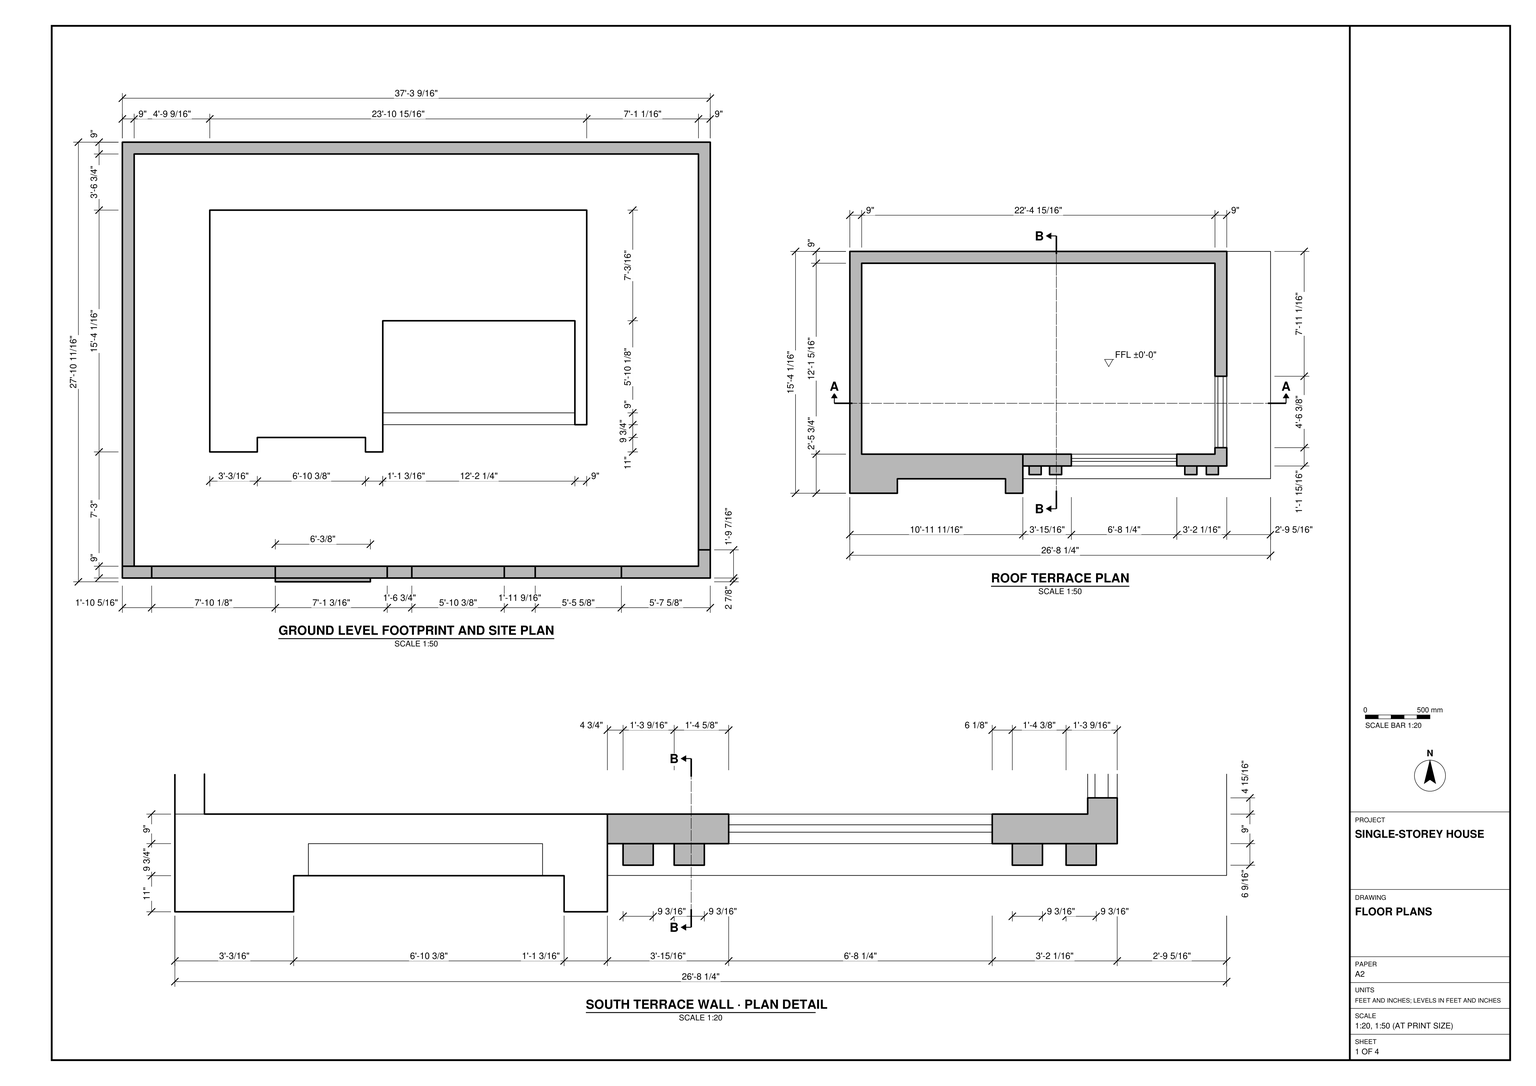
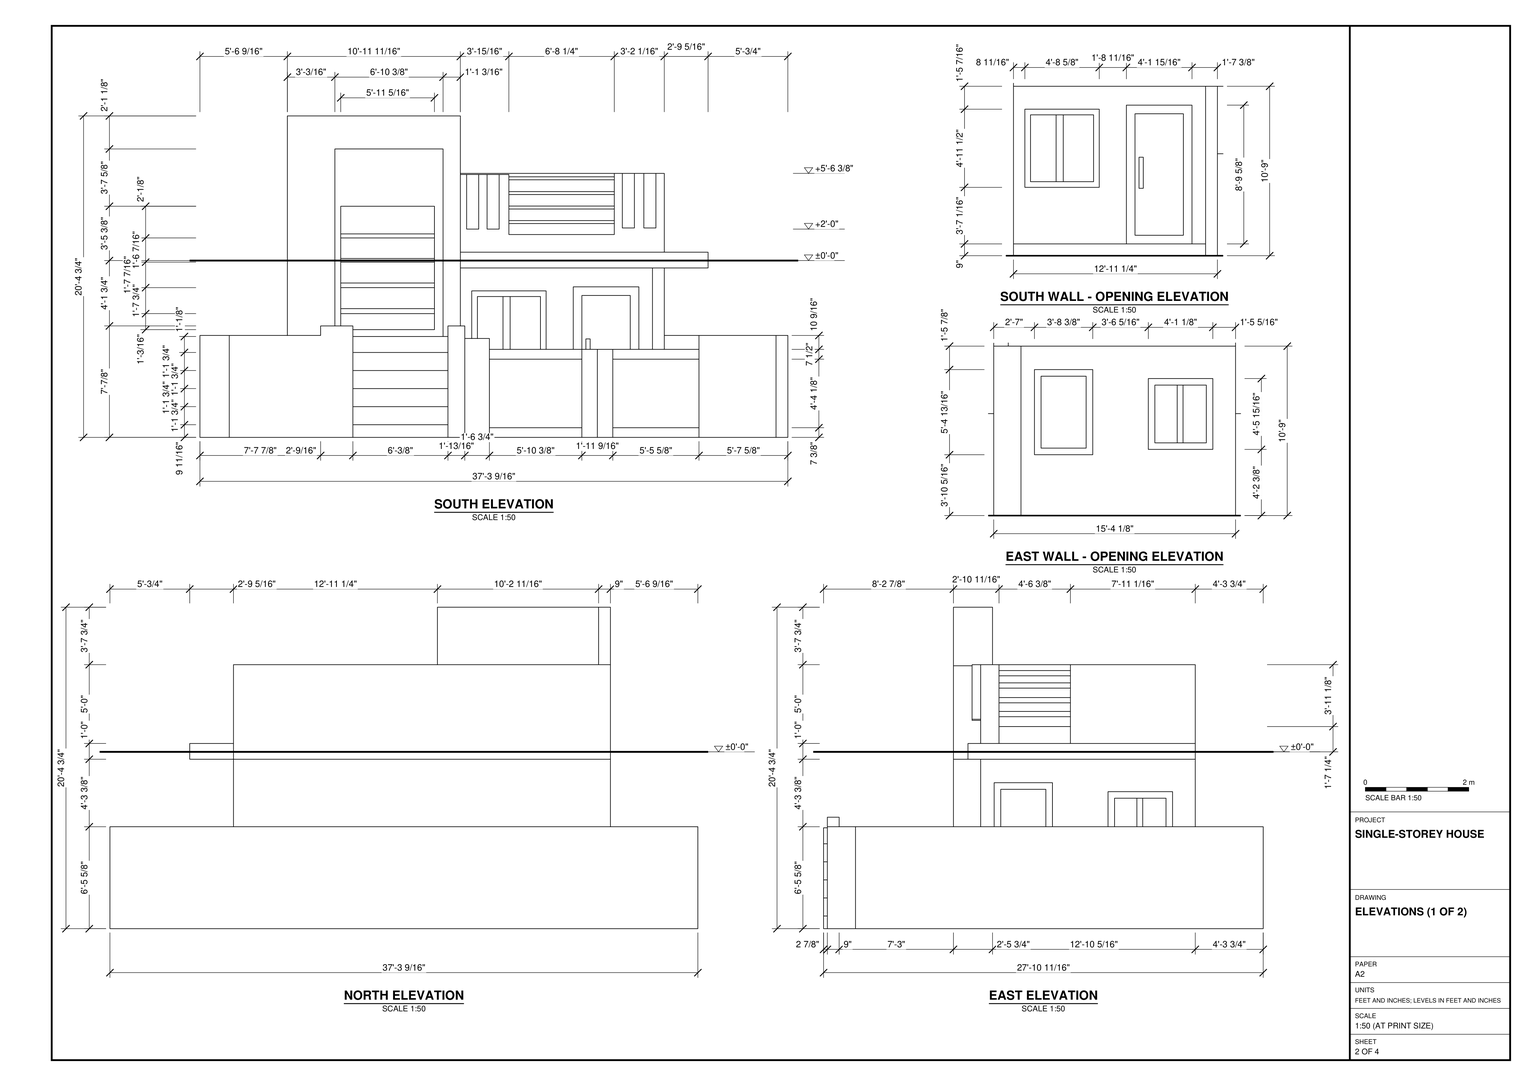
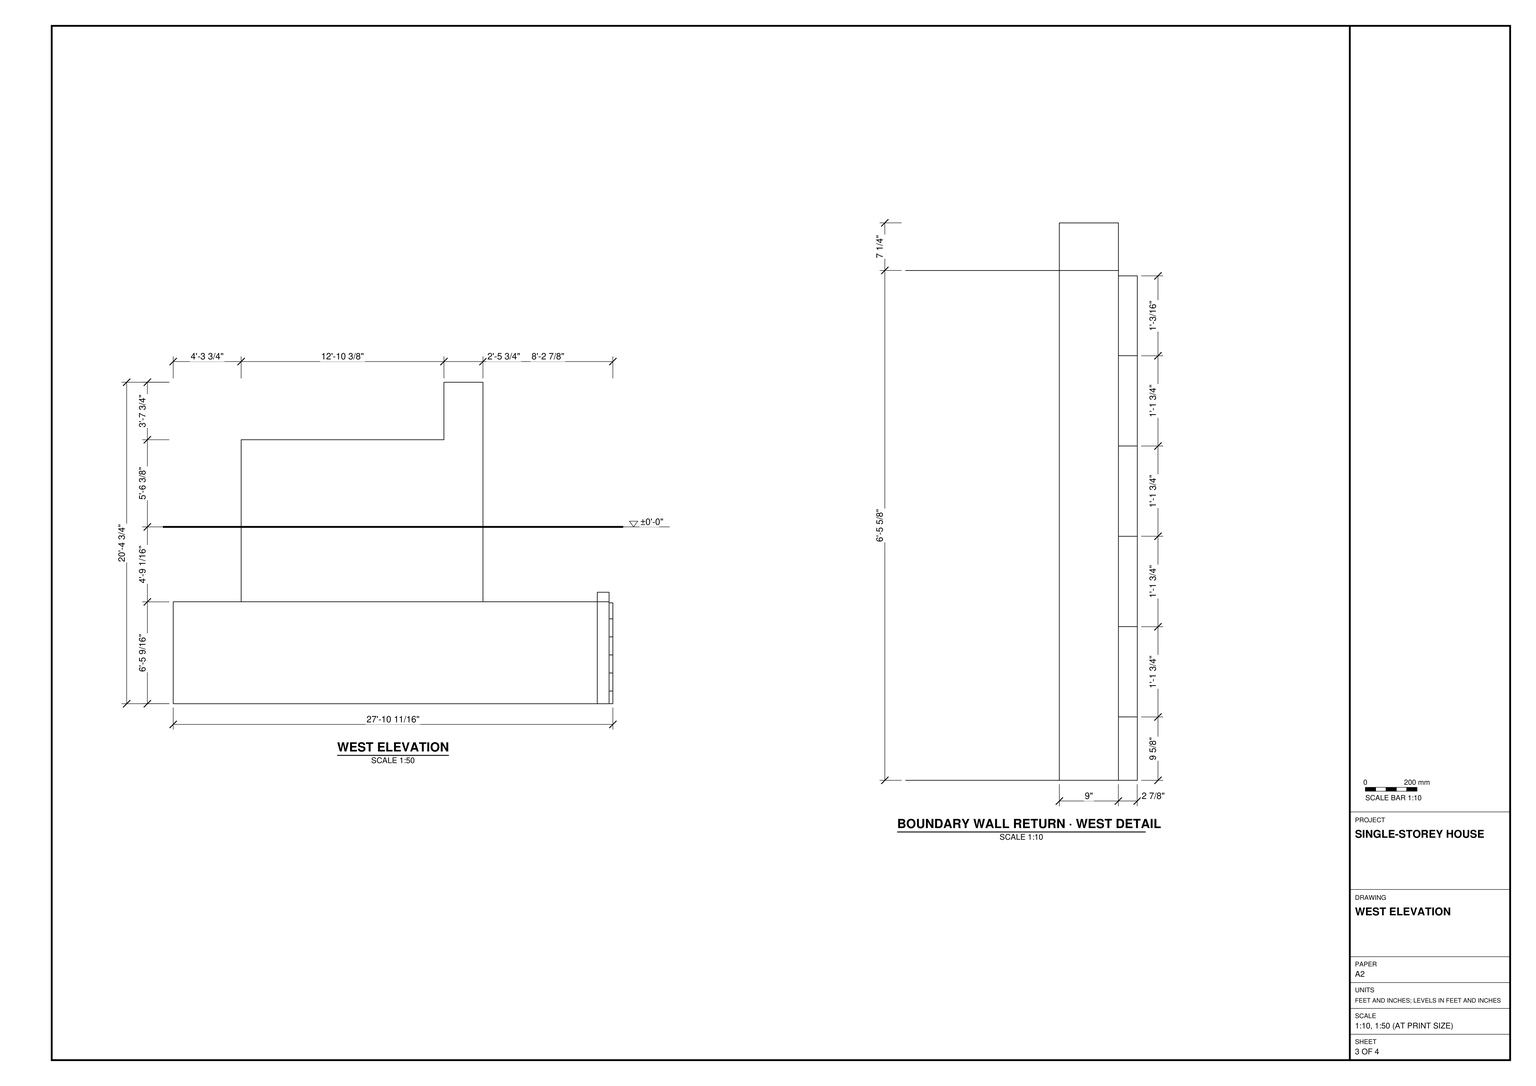
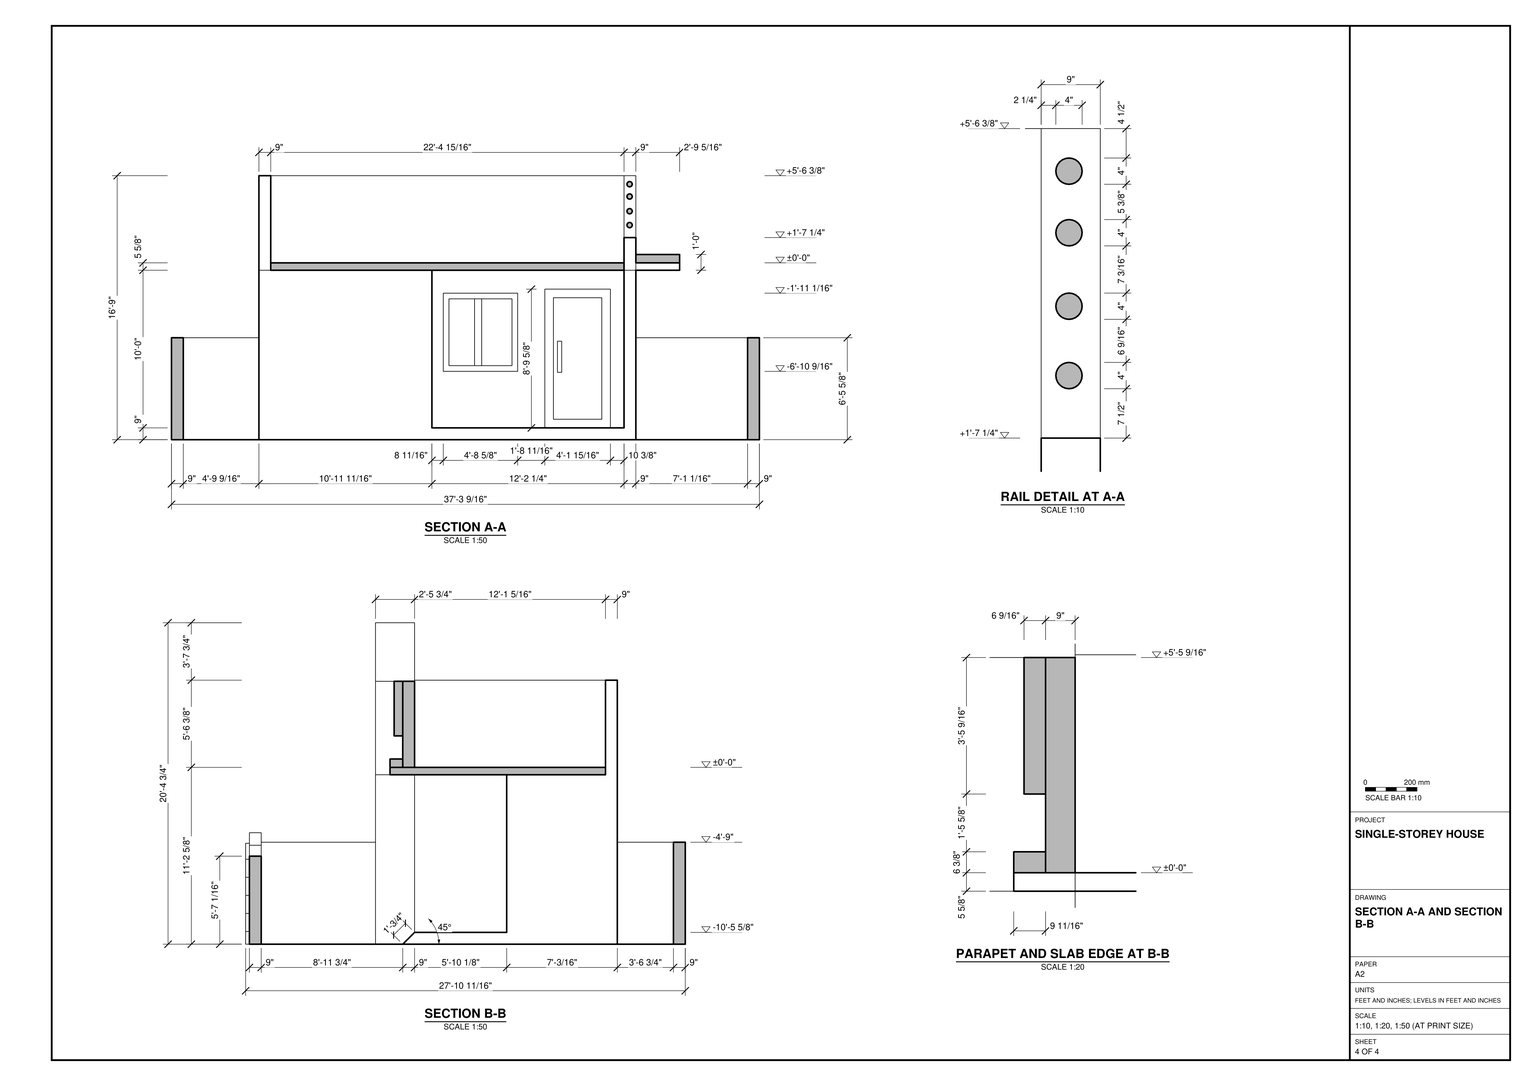
Build the single-storey house and its enclosed site in SketchUp from task_files/diagram_01.pdf. Work in feet and inches. The complete model measures 37'-3 9/16" east to west, 27'-10 11/16" north to south and 20'-4 3/4" high. Use the marked roof terrace level of ±0'-0" as the vertical reference.

Lay out the rectangular site boundary first. Position the house using the setbacks on the ground-level plan, leaving the deeper yard on the south. Trace the changes in the south face of the footprint rather than simplifying the house to a rectangle. Model the floor slab, exterior walls, framed door and window openings, and projecting flat roof slab. Use the wall thicknesses shown, including the 9" boundary walls. Follow the opening elevations for the positions of the frames, sills and window divisions.

Build the terrace parapets, the tall rectangular frame on the south facade and the horizontal infill shown in the elevations. Include the south boundary piers, recessed panels and horizontally divided gate, using the west return detail for the junction with the side wall. Keep walls, slabs and roof in separate groups or components, treat each furniture or joinery piece as a separate group or component, and use components for repeated parts. Any decor or loose items may be suitable library components. Save one SketchUp model as output_files/single_storey_house_with_walled_site_and_roof_terrace.skp.

# SketchUp Ruby script. Lengths in inches.
U = 1.inch
M = Sketchup.active_model
def pt(a) = Geom::Point3d.new(a.map { |v| v * U })
def face(e, loops, mat)
  f = e.add_face(loops[0].map { |a| pt(a) })
  loops[1..].each { |l| e.add_face(l.map { |a| pt(a) }).erase! }
  f.material = f.back_material = mat if mat
  f
end
# faces: each face lists its corners as indices into pts; further lists are holes
def faces(e, pts, list, mat = nil) = list.each { |f| face(e, (f[0].is_a?(Array) ? f : [f]).map { |l| l.map { |i| pts[i] } }, mat) }
# xy, xz, yz: faces in a plane at the given z, y or x. An outline is a flat list of corners, or four numbers for a rectangle; further outlines are holes
def ring(l) = l.size == 4 ? [[l[0], l[1]], [l[2], l[1]], [l[2], l[3]], [l[0], l[3]]] : l.each_slice(2).to_a
def flat(e, list, mat, &to3) = list.each { |f| face(e, (f[0].is_a?(Array) ? f : [f]).map { |l| ring(l).map { |u, v| to3.(u, v) } }, mat) }
def xy(e, z, list, mat = nil) = flat(e, list, mat) { |x, y| [x, y, z] }
def xz(e, y, list, mat = nil) = flat(e, list, mat) { |x, z| [x, y, z] }
def yz(e, x, list, mat = nil) = flat(e, list, mat) { |y, z| [x, y, z] }
def lines(e, pts, list) = list.each { |a, b| e.add_line(pt(pts[a]), pt(pts[b])) }
# prism: a flat outline (further loops are holes) pulled along v
def prism(e, loops, v, mat = nil)
  f = face(e, loops, mat); d = Geom::Vector3d.new(v.map { |x| x * U })
  f.pushpull(f.normal.samedirection?(d) ? d.length : -d.length)
end
def box(e, o, s, mat = nil) = prism(e, [[o, [o[0] + s[0], o[1], o[2]], [o[0] + s[0], o[1] + s[1], o[2]], [o[0], o[1] + s[1], o[2]]]], [0, 0, s[2]], mat)
def at(x, y, z, deg = 0) = Geom::Transformation.translation(pt([x, y, z])) * Geom::Transformation.rotation(ORIGIN, Z_AXIS, deg.degrees)
def axes(o, x, y, z) = Geom::Transformation.new([*x, 0, *y, 0, *z, 0, *pt(o).to_a, 1])
def part(name) = M.definitions.add(name)
# library, detail: a bought-in or finely detailed component or shape, given as its bounding box
def library(name, o, s) = part(name).tap { |d| box(d.entities, o, s) }
def detail(e, o, s) = box(e.add_group.entities, o, s)
def put(e, d, t, mat = nil) = e.add_instance(d, t).tap { |i| i.material = mat if mat }
def group(e, t, mat = nil) = e.add_group.tap { |g| g.transformation = t; g.material = mat if mat }.entities
root = M.entities
M.materials.add("[Blinds Cellular White]").color = [217, 211, 213]
M.materials.add("[Blinds Cloth Horizontal]").color = [192, 163, 85]
M.materials.add("[Blinds Roman Hobbled Blue]").color = [81, 82, 87]
M.materials.add("[Color B01]").color = [255, 216, 204]
M.materials.add("[Color D01]").color = [255, 242, 204]
M.materials.add("[Formica Beige]").color = [211, 187, 149]
M.materials.add("[Formica Graystone]").color = [149, 146, 135]
M.materials.add("[Formica Laminate Dark]").color = [50, 53, 60]
M.materials.add("[Formica Laminate Light]").color = [213, 189, 164]
M.materials.add("[Formica Speckled Grey]").color = [94, 105, 111]
M.materials.add("[Quartz Light Brown]").color = [199, 184, 152]
M.materials.add("[Quartz Light Grey]").color = [251, 251, 252]
M.materials.add("[Stone Masonry Multi]").color = [182, 175, 164]
M.materials.add("[Terrazzo Light Blue]").color = [165, 180, 191]
M.materials.add("[Terrazzo Light Blue]1").color = [196, 214, 227]
M.materials.add("[Terrazzo Tile Light]").color = [219, 217, 210]
M.materials.add("[Wood Bamboo]").color = [177, 105, 43]
M.materials.add("[Wood Floor Light]").color = [204, 176, 127]
M.materials.add("[Wood Veneer 01]").color = [71, 41, 22]
M.materials.add("[Wood Veneer 01]1").color = [120, 70, 37]
xy(root,0,[[116.43,0,188.8,2.875],[0,2.875,22.33,11.875],[22.33,2.875,116.43,11.875],[116.43,2.875,188.8,11.875],[188.8,2.875,201.63,11.875],
  [201.63,2.875,220.36,11.875],[220.36,2.875,290.74,11.875],[290.74,2.875,314.3,11.875],[314.3,2.875,379.91,11.875],[379.91,2.875,379.91,11.875,438.5625,11.875,438.5625,24.32,447.5625,24.32,447.5625,2.875],
  [0,11.875,0,334.6875,447.5625,334.6875,447.5625,24.32,438.5625,24.32,438.5625,325.6875,9,325.6875,9,11.875],[66.56,98.87,66.56,282.96,353.51,282.96,353.51,119.62,198.26,119.62,198.26,98.87,185.08,98.87,185.08,109.87,102.73,109.87,102.73,98.87]])
xy(root,0,[[[9,11.875,438.5625,325.6875],[66.56,98.87,102.73,98.87,102.73,109.87,185.08,109.87,185.08,98.87,198.26,98.87,198.26,119.62,353.51,119.62,353.51,282.96,66.56,282.96]]],"[Stone Masonry Multi]")
xy(root,9,[[198.26,128.62,344.51,198.74]],"[Terrazzo Tile Light]")
xy(root,9.66,[[116.43,0,188.8,2.875]])
xy(root,23.41,[[116.43,0,188.8,2.875]])
xy(root,37.16,[[116.43,0,188.8,2.875]])
xy(root,50.91,[[116.43,0,188.8,2.875]])
xy(root,64.66,[[116.43,0,188.8,2.875]])
xy(root,67.04,[[220.36,2.875,290.74,11.875],[314.3,2.875,379.91,11.875]],"[Formica Beige]")
xy(root,67.04,[[290.74,2.875,314.3,11.875]],"[Formica Speckled Grey]")
xy(root,75.3125,[[201.63,2.875,220.36,11.875]],"[Formica Speckled Grey]")
xy(root,76.8125,[[116.43,2.875,188.8,11.875]],"[Color D01]")
xy(root,76.8125,[[116.43,0,188.8,2.875]],"[Terrazzo Light Blue]")
xy(root,77.625,[[22.33,2.875,91.89,11.875]],"[Color D01]")
xy(root,77.625,[[0,11.875,9,11.875,9,325.6875,438.5625,325.6875,438.5625,24.32,447.5625,24.32,447.5625,334.6875,0,334.6875]],"[Formica Laminate Light]")
xy(root,77.625,[[0,2.875,22.33,11.875],[379.91,2.875,438.5625,11.875],[438.5625,2.875,447.5625,24.32]],"[Formica Speckled Grey]")
xy(root,82.04,[[107.2,109.87,178.52,119.62]],"[Terrazzo Light Blue]1")
xy(root,84.875,[[91.89,2.875,116.43,11.875],[188.8,2.875,201.63,11.875]],"[Color D01]")
xy(root,129,[[75.56,128.62,198.26,198.74],[75.56,198.74,344.51,273.96]])
xy(root,129,[[198.26,109.93,198.26,198.74,344.51,198.74,344.51,119.62,386.82,119.62,386.82,109.93],[353.51,119.62,386.82,282.96]],"[Formica Beige]")
xy(root,134.625,[[198.26,109.93,386.82,119.62],[198.26,119.62,235.19,128.62],[235.19,119.62,315.44,128.62],[315.44,119.62,344.51,128.62],[344.51,119.62,353.51,133.56],
  [353.51,119.62,386.82,282.96]])
xy(root,134.625,[[75.56,128.62,344.51,273.96]],"[Formica Graystone]")
xy(root,141,[[198.26,109.93,386.82,109.93,386.82,282.96,353.51,282.96,353.51,119.62,198.26,119.62]],"[Formica Beige]")
xy(root,153.875,[[344.51,133.56,353.51,187.91]],"[Terrazzo Light Blue]1")
xy(root,154.4375,[[235.19,119.62,315.44,128.62]],"[Terrazzo Light Blue]1")
xy(root,158.6,[[203.03,113.05,212.22,119.62],[218.59,113.05,227.78,119.62]],"[Color B01]")
xy(root,159.4375,[[321.56,113.05,330.74,119.62],[337.93,113.05,347.12,119.62]],"[Color B01]")
xy(root,175.98,[[107.2,109.87,178.52,119.62]],"[Terrazzo Light Blue]1")
xy(root,200.16,[[203.03,113.05,212.22,119.62],[218.59,113.05,227.78,119.62]],"[Color B01]")
xy(root,200.16,[[198.26,119.62,235.19,128.62]],"[Terrazzo Light Blue]1")
xy(root,201,[[321.56,113.05,330.74,119.62],[337.93,113.05,347.12,119.62]],"[Color B01]")
xy(root,201,[[66.56,128.62,75.56,128.62,75.56,273.96,344.51,273.96,344.51,187.91,353.51,187.91,353.51,282.96,66.56,282.96]],"[Terrazzo Light Blue]")
xy(root,201,[[315.44,119.62,353.51,119.62,353.51,133.56,344.51,133.56,344.51,128.62,315.44,128.62]],"[Terrazzo Light Blue]1")
xy(root,219.6,[[102.73,98.87,185.08,109.87]],"[Formica Speckled Grey]")
xy(root,244.75,[[66.56,98.87,198.26,128.62]],"[Formica Speckled Grey]")
xz(root,0,[[116.43,0,188.8,9.66],[116.43,9.66,188.8,23.41],[116.43,23.41,188.8,37.16],[116.43,37.16,188.8,50.91],[116.43,50.91,188.8,64.66],
  [116.43,64.66,188.8,76.8125]],"[Terrazzo Light Blue]")
xz(root,2.875,[[116.43,0,188.8,9.66],[116.43,9.66,188.8,23.41],[116.43,23.41,188.8,37.16],[116.43,37.16,188.8,50.91],[116.43,50.91,188.8,64.66],
  [116.43,64.66,188.8,76.8125]])
xz(root,2.875,[[22.33,0,116.43,0,116.43,84.875,91.89,84.875,91.89,77.625,22.33,77.625],[188.8,0,201.63,84.875],[438.5625,0,447.5625,77.625]],"[Color D01]")
xz(root,2.875,[[220.36,0,290.74,7.38],[314.3,0,379.91,7.38],[220.36,59.53,290.74,67.04],[314.3,59.53,379.91,67.04]],"[Formica Beige]")
xz(root,2.875,[[0,0,22.33,77.625],[201.63,0,220.36,75.3125],[290.74,0,302.52,67.04],[302.52,0,314.3,67.04],[379.91,0,438.5625,77.625],
  [220.36,7.38,290.74,59.53],[314.3,7.38,379.91,59.53]],"[Formica Speckled Grey]")
xz(root,11.875,[[0,0,9,77.625]])
xz(root,11.875,[[220.36,0,290.74,67.04],[314.3,0,379.91,67.04]],"[Formica Beige]")
xz(root,11.875,[[9,0,22.33,77.625],[22.33,0,22.33,77.625,91.89,77.625,91.89,84.875,116.43,84.875,116.43,0],[116.43,0,188.8,76.8125],[188.8,0,201.63,84.875]],"[Formica Laminate Light]")
xz(root,11.875,[[201.63,0,220.36,75.3125],[290.74,0,314.3,67.04],[379.91,0,438.5625,77.625]],"[Formica Speckled Grey]")
xz(root,24.32,[[438.5625,0,447.5625,77.625]])
xz(root,98.87,[[66.56,0,102.73,0,102.73,219.6,185.08,219.6,185.08,0,198.26,0,198.26,244.75,66.56,244.75]],"[Formica Speckled Grey]")
xz(root,109.87,[[[102.73,0,185.08,219.6],[107.2,82.04,178.52,175.98]]],"[Terrazzo Light Blue]")
xz(root,109.93,[[198.26,129,386.82,134.625],[198.26,134.625,386.82,141]],"[Quartz Light Grey]")
xz(root,113.05,[[203.03,158.6,212.22,200.16],[218.59,158.6,227.78,200.16],[321.56,159.4375,330.74,201],[337.93,159.4375,347.12,201]],"[Color B01]")
xz(root,119.62,[[198.26,134.625,235.19,141],[235.19,134.625,315.44,141],[315.44,134.625,344.51,141],[344.51,134.625,353.51,141],[203.03,158.6,212.22,200.16],
  [218.59,158.6,227.78,200.16],[321.56,159.4375,330.74,201],[337.93,159.4375,347.12,201]])
xz(root,119.62,[[107.2,82.04,178.52,94.23],[107.2,98.03,178.52,114.01],[107.2,117.54,178.52,133.42],[107.2,136.2,178.52,151.85],[107.2,154.93,178.52,175.98]],"[Blinds Roman Hobbled Blue]")
xz(root,119.62,[[107.2,94.23,178.52,98.03],[107.2,114.01,178.52,117.54],[107.2,133.42,178.52,136.2],[107.2,151.85,178.52,154.93]],"[Color B01]")
xz(root,119.62,[[344.51,0,353.51,129],[198.26,141,353.51,141,353.51,201,347.12,201,347.12,159.4375,337.93,159.4375,337.93,201,330.74,201,330.74,159.4375,321.56,159.4375,321.56,201,315.44,201,315.44,154.4375,235.19,154.4375,235.19,200.16,227.78,200.16,227.78,158.6,218.59,158.6,218.59,200.16,212.22,200.16,212.22,158.6,203.03,158.6,203.03,200.16,198.26,200.16]],"[Terrazzo Light Blue]")
xz(root,128.62,[[75.56,129,198.26,134.625]])
xz(root,128.62,[[75.56,134.625,198.26,244.75],[198.26,134.625,235.19,200.16],[235.19,134.625,315.44,154.4375],[315.44,134.625,344.51,201],[66.56,201,75.56,244.75]],"[Terrazzo Light Blue]1")
xz(root,133.56,[[344.51,134.625,353.51,153.875],[[344.51,153.875,353.51,201],[348.74,192.52,348.22,192.59,347.74,192.79,347.33,193.1,347.01,193.52,346.81,194,346.74,194.52,346.81,195.04,347.01,195.52,347.33,195.93,347.74,196.25,348.22,196.45,348.74,196.52,349.26,196.45,349.74,196.25,350.15,195.93,350.47,195.52,350.67,195.04,350.74,194.52,350.67,194,350.47,193.52,350.15,193.1,349.74,192.79,349.26,192.59],[348.74,183.14,348.22,183.21,347.74,183.41,347.33,183.73,347.01,184.14,346.81,184.625,346.74,185.14,346.81,185.66,347.01,186.14,347.33,186.56,347.74,186.875,348.22,187.07,348.74,187.14,349.26,187.07,349.74,186.875,350.15,186.56,350.47,186.14,350.67,185.66,350.74,185.14,350.67,184.625,350.47,184.14,350.15,183.73,349.74,183.41,349.26,183.21],[348.74,171.96,348.22,172.02,347.74,172.22,347.33,172.54,347.01,172.96,346.81,173.4375,346.74,173.96,346.81,174.47,347.01,174.96,347.33,175.37,347.74,175.6875,348.22,175.89,348.74,175.96,349.26,175.89,349.74,175.6875,350.15,175.37,350.47,174.96,350.67,174.47,350.74,173.96,350.67,173.4375,350.47,172.96,350.15,172.54,349.74,172.22,349.26,172.02],[348.74,161.39,348.22,161.46,347.74,161.66,347.33,161.98,347.01,162.39,346.81,162.875,346.74,163.39,346.81,163.91,347.01,164.39,347.33,164.81,347.74,165.125,348.22,165.32,348.74,165.39,349.26,165.32,349.74,165.125,350.15,164.81,350.47,164.39,350.67,163.91,350.74,163.39,350.67,162.875,350.47,162.39,350.15,161.98,349.74,161.66,349.26,161.46]]])
xz(root,187.91,[[348.74,161.39,348.22,161.46,347.74,161.66,347.33,161.98,347.01,162.39,346.81,162.875,346.74,163.39,346.81,163.91,347.01,164.39,347.33,164.81,347.74,165.125,348.22,165.32,348.74,165.39,349.26,165.32,349.74,165.125,350.15,164.81,350.47,164.39,350.67,163.91,350.74,163.39,350.67,162.875,350.47,162.39,350.15,161.98,349.74,161.66,349.26,161.46],[348.74,171.96,348.22,172.02,347.74,172.22,347.33,172.54,347.01,172.96,346.81,173.4375,346.74,173.96,346.81,174.47,347.01,174.96,347.33,175.37,347.74,175.6875,348.22,175.89,348.74,175.96,349.26,175.89,349.74,175.6875,350.15,175.37,350.47,174.96,350.67,174.47,350.74,173.96,350.67,173.4375,350.47,172.96,350.15,172.54,349.74,172.22,349.26,172.02],[348.74,183.14,348.22,183.21,347.74,183.41,347.33,183.73,347.01,184.14,346.81,184.625,346.74,185.14,346.81,185.66,347.01,186.14,347.33,186.56,347.74,186.875,348.22,187.07,348.74,187.14,349.26,187.07,349.74,186.875,350.15,186.56,350.47,186.14,350.67,185.66,350.74,185.14,350.67,184.625,350.47,184.14,350.15,183.73,349.74,183.41,349.26,183.21],[348.74,192.52,348.22,192.59,347.74,192.79,347.33,193.1,347.01,193.52,346.81,194,346.74,194.52,346.81,195.04,347.01,195.52,347.33,195.93,347.74,196.25,348.22,196.45,348.74,196.52,349.26,196.45,349.74,196.25,350.15,195.93,350.47,195.52,350.67,195.04,350.74,194.52,350.67,194,350.47,193.52,350.15,193.1,349.74,192.79,349.26,192.59]])
xz(root,187.91,[[[344.51,153.875,353.51,201],[348.74,192.52,348.22,192.59,347.74,192.79,347.33,193.1,347.01,193.52,346.81,194,346.74,194.52,346.81,195.04,347.01,195.52,347.33,195.93,347.74,196.25,348.22,196.45,348.74,196.52,349.26,196.45,349.74,196.25,350.15,195.93,350.47,195.52,350.67,195.04,350.74,194.52,350.67,194,350.47,193.52,350.15,193.1,349.74,192.79,349.26,192.59],[348.74,161.39,348.22,161.46,347.74,161.66,347.33,161.98,347.01,162.39,346.81,162.875,346.74,163.39,346.81,163.91,347.01,164.39,347.33,164.81,347.74,165.125,348.22,165.32,348.74,165.39,349.26,165.32,349.74,165.125,350.15,164.81,350.47,164.39,350.67,163.91,350.74,163.39,350.67,162.875,350.47,162.39,350.15,161.98,349.74,161.66,349.26,161.46],[348.74,183.14,348.22,183.21,347.74,183.41,347.33,183.73,347.01,184.14,346.81,184.625,346.74,185.14,346.81,185.66,347.01,186.14,347.33,186.56,347.74,186.875,348.22,187.07,348.74,187.14,349.26,187.07,349.74,186.875,350.15,186.56,350.47,186.14,350.67,185.66,350.74,185.14,350.67,184.625,350.47,184.14,350.15,183.73,349.74,183.41,349.26,183.21],[348.74,171.96,348.22,172.02,347.74,172.22,347.33,172.54,347.01,172.96,346.81,173.4375,346.74,173.96,346.81,174.47,347.01,174.96,347.33,175.37,347.74,175.6875,348.22,175.89,348.74,175.96,349.26,175.89,349.74,175.6875,350.15,175.37,350.47,174.96,350.67,174.47,350.74,173.96,350.67,173.4375,350.47,172.96,350.15,172.54,349.74,172.22,349.26,172.02]]],"[Terrazzo Light Blue]1")
xz(root,198.74,[[211.23,56.36,230.72,107.24],[236.15,56.36,259.23,107.24]],"[Blinds Roman Hobbled Blue]")
xz(root,198.74,[[[198.26,9,284.21,9,284.21,114.625,334.14,114.625,334.14,9,344.51,9,344.51,129,198.26,129],[206.92,52.05,263.54,111.55]]],"[Terrazzo Light Blue]")
xz(root,198.74,[[[290.77,15.5625,327.58,108.0625],[293.8125,51.3,297.0625,74.99]]],"[Wood Bamboo]")
xz(root,198.74,[[293.8125,51.3,297.0625,74.99]],"[Wood Floor Light]")
xz(root,198.74,[[[284.21,9,334.14,114.625],[290.77,15.5625,327.58,108.0625]],[[206.92,52.05,263.54,111.55],[211.23,56.36,259.23,107.24]],[230.72,56.36,236.15,107.24]],"[Wood Veneer 01]")
xz(root,273.96,[[75.56,129,344.51,134.625]])
xz(root,273.96,[[75.56,134.625,344.51,201]],"[Formica Graystone]")
xz(root,282.96,[[353.51,129,386.82,134.625],[353.51,134.625,386.82,141]],"[Quartz Light Grey]")
xz(root,282.96,[[66.56,0,353.51,129],[66.56,129,353.51,201]],"[Terrazzo Light Blue]")
xz(root,325.6875,[[9,0,438.5625,77.625]],"[Formica Laminate Light]")
xz(root,334.6875,[[0,0,447.5625,77.625]],"[Color D01]")
yz(root,0,[[11.875,0,334.6875,77.625]],"[Color D01]")
yz(root,0,[[2.875,0,11.875,77.625]],"[Formica Speckled Grey]")
yz(root,9,[[11.875,0,325.6875,77.625]],"[Formica Laminate Light]")
yz(root,22.33,[[2.875,0,11.875,77.625]])
yz(root,66.56,[[98.87,0,98.87,244.75,128.62,244.75,128.62,201,282.96,201,282.96,0]],"[Terrazzo Light Blue]")
yz(root,75.56,[[128.62,129,198.74,134.625],[198.74,129,273.96,134.625]])
yz(root,75.56,[[128.62,134.625,273.96,201]],"[Formica Graystone]")
yz(root,91.89,[[2.875,77.625,11.875,84.875]])
yz(root,102.73,[[98.87,0,109.87,219.6]],"[Formica Speckled Grey]")
yz(root,107.2,[[109.87,82.04,119.62,175.98]],"[Terrazzo Light Blue]1")
yz(root,116.43,[[2.875,0,11.875,76.8125],[2.875,76.8125,11.875,84.875]])
yz(root,116.43,[[0,0,2.875,9.66],[0,9.66,2.875,23.41],[0,23.41,2.875,37.16],[0,37.16,2.875,50.91],[0,50.91,2.875,64.66],
  [0,64.66,2.875,76.8125]],"[Terrazzo Light Blue]")
yz(root,178.52,[[109.87,82.04,119.62,175.98]],"[Terrazzo Light Blue]1")
yz(root,185.08,[[98.87,0,109.87,219.6]],"[Formica Speckled Grey]")
yz(root,188.8,[[2.875,76.8125,11.875,84.875]],"[Color D01]")
yz(root,188.8,[[0,0,2.875,9.66],[0,9.66,2.875,23.41],[0,23.41,2.875,37.16],[0,37.16,2.875,50.91],[0,50.91,2.875,64.66],
  [0,64.66,2.875,76.8125]],"[Terrazzo Light Blue]")
yz(root,198.26,[[109.93,129,128.62,134.625],[109.93,134.625,119.62,141],[119.62,134.625,128.62,200.16]])
yz(root,198.26,[[98.87,129,109.93,129,109.93,141,119.62,141,119.62,200.16,98.87,200.16],[98.87,200.16,128.62,244.75]],"[Formica Speckled Grey]")
yz(root,198.26,[[98.87,0,119.62,0,128.62,9,128.62,129,98.87,129],[128.62,9,198.74,129]],"[Terrazzo Light Blue]")
yz(root,201.63,[[2.875,0,11.875,75.3125]])
yz(root,201.63,[[2.875,75.3125,11.875,84.875]],"[Quartz Light Brown]")
yz(root,203.03,[[113.05,158.6,119.62,200.16]],"[Color B01]")
yz(root,212.22,[[113.05,158.6,119.62,200.16]],"[Color B01]")
yz(root,218.59,[[113.05,158.6,119.62,200.16]],"[Color B01]")
yz(root,220.36,[[2.875,0,11.875,67.04]])
yz(root,220.36,[[2.875,67.04,11.875,75.3125]],"[Formica Speckled Grey]")
yz(root,227.78,[[113.05,158.6,119.62,200.16]],"[Color B01]")
yz(root,235.19,[[[119.62,154.4375,128.62,200.16],[124.23,196.13,123.9375,196.17,123.67,196.28,123.43,196.46,123.26,196.69,123.14,196.96,123.1,197.25,123.14,197.54,123.26,197.81,123.43,198.05,123.67,198.23,123.9375,198.34,124.23,198.38,124.52,198.34,124.79,198.23,125.03,198.05,125.2,197.81,125.32,197.54,125.35,197.25,125.32,196.96,125.2,196.69,125.03,196.46,124.79,196.28,124.52,196.17],[124.23,184.88,123.9375,184.92,123.67,185.03,123.43,185.21,123.26,185.44,123.14,185.71,123.1,186,123.14,186.29,123.26,186.56,123.43,186.8,123.67,186.98,123.9375,187.09,124.23,187.13,124.52,187.09,124.79,186.98,125.03,186.8,125.2,186.56,125.32,186.29,125.35,186,125.32,185.71,125.2,185.44,125.03,185.21,124.79,185.03,124.52,184.92],[124.23,173.88,123.9375,173.92,123.67,174.03,123.43,174.21,123.26,174.44,123.14,174.71,123.1,175,123.14,175.29,123.26,175.56,123.43,175.8,123.67,175.98,123.9375,176.09,124.23,176.13,124.52,176.09,124.79,175.98,125.03,175.8,125.2,175.56,125.32,175.29,125.35,175,125.32,174.71,125.2,174.44,125.03,174.21,124.79,174.03,124.52,173.92],[124.23,162.81,123.9375,162.85,123.67,162.97,123.43,163.14,123.26,163.38,123.14,163.65,123.1,163.94,123.14,164.23,123.26,164.5,123.43,164.74,123.67,164.91,123.9375,165.03,124.23,165.06,124.52,165.03,124.79,164.91,125.03,164.74,125.2,164.5,125.32,164.23,125.35,163.94,125.32,163.65,125.2,163.38,125.03,163.14,124.79,162.97,124.52,162.85]]],"[Terrazzo Light Blue]1")
yz(root,290.74,[[2.875,0,11.875,67.04]])
yz(root,314.3,[[2.875,0,11.875,67.04]])
yz(root,315.44,[[124.23,162.81,124.52,162.85,124.79,162.97,125.03,163.14,125.2,163.38,125.32,163.65,125.35,163.94,125.32,164.23,125.2,164.5,125.03,164.74,124.79,164.91,124.52,165.03,124.23,165.06,123.9375,165.03,123.67,164.91,123.43,164.74,123.26,164.5,123.14,164.23,123.1,163.94,123.14,163.65,123.26,163.38,123.43,163.14,123.67,162.97,123.9375,162.85],[124.23,173.88,124.52,173.92,124.79,174.03,125.03,174.21,125.2,174.44,125.32,174.71,125.35,175,125.32,175.29,125.2,175.56,125.03,175.8,124.79,175.98,124.52,176.09,124.23,176.13,123.9375,176.09,123.67,175.98,123.43,175.8,123.26,175.56,123.14,175.29,123.1,175,123.14,174.71,123.26,174.44,123.43,174.21,123.67,174.03,123.9375,173.92],[124.23,184.88,124.52,184.92,124.79,185.03,125.03,185.21,125.2,185.44,125.32,185.71,125.35,186,125.32,186.29,125.2,186.56,125.03,186.8,124.79,186.98,124.52,187.09,124.23,187.13,123.9375,187.09,123.67,186.98,123.43,186.8,123.26,186.56,123.14,186.29,123.1,186,123.14,185.71,123.26,185.44,123.43,185.21,123.67,185.03,123.9375,184.92],[124.23,196.13,124.52,196.17,124.79,196.28,125.03,196.46,125.2,196.69,125.32,196.96,125.35,197.25,125.32,197.54,125.2,197.81,125.03,198.05,124.79,198.23,124.52,198.34,124.23,198.38,123.9375,198.34,123.67,198.23,123.43,198.05,123.26,197.81,123.14,197.54,123.1,197.25,123.14,196.96,123.26,196.69,123.43,196.46,123.67,196.28,123.9375,196.17]])
yz(root,315.44,[[[119.62,154.4375,128.62,201],[124.23,196.13,124.52,196.17,124.79,196.28,125.03,196.46,125.2,196.69,125.32,196.96,125.35,197.25,125.32,197.54,125.2,197.81,125.03,198.05,124.79,198.23,124.52,198.34,124.23,198.38,123.9375,198.34,123.67,198.23,123.43,198.05,123.26,197.81,123.14,197.54,123.1,197.25,123.14,196.96,123.26,196.69,123.43,196.46,123.67,196.28,123.9375,196.17],[124.23,162.81,124.52,162.85,124.79,162.97,125.03,163.14,125.2,163.38,125.32,163.65,125.35,163.94,125.32,164.23,125.2,164.5,125.03,164.74,124.79,164.91,124.52,165.03,124.23,165.06,123.9375,165.03,123.67,164.91,123.43,164.74,123.26,164.5,123.14,164.23,123.1,163.94,123.14,163.65,123.26,163.38,123.43,163.14,123.67,162.97,123.9375,162.85],[124.23,184.88,124.52,184.92,124.79,185.03,125.03,185.21,125.2,185.44,125.32,185.71,125.35,186,125.32,186.29,125.2,186.56,125.03,186.8,124.79,186.98,124.52,187.09,124.23,187.13,123.9375,187.09,123.67,186.98,123.43,186.8,123.26,186.56,123.14,186.29,123.1,186,123.14,185.71,123.26,185.44,123.43,185.21,123.67,185.03,123.9375,184.92],[124.23,173.88,124.52,173.92,124.79,174.03,125.03,174.21,125.2,174.44,125.32,174.71,125.35,175,125.32,175.29,125.2,175.56,125.03,175.8,124.79,175.98,124.52,176.09,124.23,176.13,123.9375,176.09,123.67,175.98,123.43,175.8,123.26,175.56,123.14,175.29,123.1,175,123.14,174.71,123.26,174.44,123.43,174.21,123.67,174.03,123.9375,173.92]]],"[Terrazzo Light Blue]1")
yz(root,321.56,[[113.05,159.4375,119.62,201]],"[Color B01]")
yz(root,330.74,[[113.05,159.4375,119.62,201]],"[Color B01]")
yz(root,337.93,[[113.05,159.4375,119.62,201]],"[Color B01]")
yz(root,344.51,[[119.62,129,198.74,134.625],[198.74,129,273.96,134.625]])
yz(root,344.51,[[133.56,134.625,187.91,153.875],[187.91,134.625,273.96,201]],"[Formica Graystone]")
yz(root,344.51,[[119.62,0,119.62,129,128.62,129,128.62,9],[128.62,9,198.74,129]],"[Terrazzo Light Blue]")
yz(root,344.51,[[128.62,134.625,133.56,201]],"[Terrazzo Light Blue]1")
yz(root,347.12,[[113.05,159.4375,119.62,201]],"[Color B01]")
yz(root,353.51,[[119.62,134.625,133.56,141],[133.56,134.625,187.91,141],[187.91,134.625,282.96,141]])
yz(root,353.51,[[221.53,55.36,238.53,99.34],[242.97,55.36,260.7,99.34]],"[Blinds Cellular White]")
yz(root,353.51,[[134.9,51.36,169.22,106.12]],"[Blinds Cloth Horizontal]")
yz(root,353.51,[[[119.62,0,282.96,129],[129.87,46.33,174.24,111.14],[216.55,50.38,265.67,104.32]],[119.62,141,133.56,201],[133.56,141,187.91,153.875],[187.91,141,282.96,201]],"[Terrazzo Light Blue]")
yz(root,353.51,[[[129.87,46.33,174.24,111.14],[134.9,51.36,169.22,106.12]]],"[Wood Bamboo]")
yz(root,353.51,[[[216.55,50.38,265.67,104.32],[221.53,55.36,260.7,99.34]],[238.53,55.36,242.97,99.34]],"[Wood Veneer 01]1")
yz(root,379.91,[[2.875,0,11.875,67.04]])
yz(root,379.91,[[2.875,67.04,11.875,77.625]],"[Formica Speckled Grey]")
yz(root,386.82,[[109.93,129,282.96,134.625],[109.93,134.625,282.96,141]],"[Quartz Light Grey]")
yz(root,438.5625,[[11.875,0,24.32,77.625],[24.32,0,325.6875,77.625]],"[Formica Laminate Light]")
yz(root,447.5625,[[24.32,0,334.6875,77.625]],"[Color D01]")
yz(root,447.5625,[[2.875,0,24.32,77.625]],"[Formica Speckled Grey]")
p = [[344.51,119.62,0],[344.51,128.62,9],[198.26,128.62,9],[198.26,119.62,0],[348.22,187.91,161.46],[348.74,187.91,161.39],
  [348.74,133.56,161.39],[348.22,133.56,161.46],[349.26,187.91,161.46],[349.26,133.56,161.46],[347.74,187.91,161.66],[347.74,133.56,161.66],
  [349.74,187.91,161.66],[349.74,133.56,161.66],[347.33,187.91,161.98],[347.33,133.56,161.98],[350.15,187.91,161.98],[350.15,133.56,161.98],
  [347.01,187.91,162.39],[347.01,133.56,162.39],[350.47,187.91,162.39],[350.47,133.56,162.39],[346.81,187.91,162.875],[346.81,133.56,162.875],
  [350.67,187.91,162.875],[350.67,133.56,162.875],[315.44,124.23,162.81],[315.44,123.9375,162.85],[235.19,123.9375,162.85],[235.19,124.23,162.81],
  [315.44,124.52,162.85],[235.19,124.52,162.85],[315.44,123.67,162.97],[235.19,123.67,162.97],[315.44,124.79,162.97],[235.19,124.79,162.97],
  [346.74,187.91,163.39],[346.74,133.56,163.39],[350.74,187.91,163.39],[350.74,133.56,163.39],[315.44,123.43,163.14],[235.19,123.43,163.14],
  [315.44,125.03,163.14],[235.19,125.03,163.14],[315.44,123.26,163.38],[235.19,123.26,163.38],[315.44,125.2,163.38],[235.19,125.2,163.38],
  [315.44,123.14,163.65],[235.19,123.14,163.65],[315.44,125.32,163.65],[235.19,125.32,163.65],[346.81,187.91,163.91],[346.81,133.56,163.91],
  [350.67,187.91,163.91],[350.67,133.56,163.91],[315.44,123.1,163.94],[235.19,123.1,163.94],[315.44,125.35,163.94],[235.19,125.35,163.94],
  [315.44,123.14,164.23],[235.19,123.14,164.23],[315.44,125.32,164.23],[235.19,125.32,164.23],[347.01,187.91,164.39],[347.01,133.56,164.39],
  [350.47,187.91,164.39],[350.47,133.56,164.39],[315.44,123.26,164.5],[235.19,123.26,164.5],[315.44,125.2,164.5],[235.19,125.2,164.5],
  [347.33,187.91,164.81],[347.33,133.56,164.81],[350.15,187.91,164.81],[350.15,133.56,164.81],[315.44,123.43,164.74],[235.19,123.43,164.74],
  [315.44,125.03,164.74],[235.19,125.03,164.74],[315.44,123.67,164.91],[235.19,123.67,164.91],[315.44,124.79,164.91],[235.19,124.79,164.91],
  [347.74,187.91,165.125],[347.74,133.56,165.125],[349.74,187.91,165.125],[349.74,133.56,165.125],[315.44,123.9375,165.03],[235.19,123.9375,165.03],
  [315.44,124.52,165.03],[235.19,124.52,165.03],[315.44,124.23,165.06],[235.19,124.23,165.06],[348.22,187.91,165.32],[348.22,133.56,165.32],
  [349.26,187.91,165.32],[349.26,133.56,165.32],[348.74,187.91,165.39],[348.74,133.56,165.39],[347.74,187.91,172.22],[348.22,187.91,172.02],
  [348.22,133.56,172.02],[347.74,133.56,172.22],[348.74,187.91,171.96],[348.74,133.56,171.96],[349.26,187.91,172.02],[349.26,133.56,172.02],
  [349.74,187.91,172.22],[349.74,133.56,172.22],[347.33,187.91,172.54],[347.33,133.56,172.54],[350.15,187.91,172.54],[350.15,133.56,172.54],
  [347.01,187.91,172.96],[347.01,133.56,172.96],[350.47,187.91,172.96],[350.47,133.56,172.96],[346.81,187.91,173.4375],[346.81,133.56,173.4375],
  [350.67,187.91,173.4375],[350.67,133.56,173.4375],[346.74,187.91,173.96],[346.74,133.56,173.96],[350.74,187.91,173.96],[350.74,133.56,173.96],
  [315.44,123.9375,173.92],[315.44,123.67,174.03],[235.19,123.67,174.03],[235.19,123.9375,173.92],[315.44,124.23,173.88],[235.19,124.23,173.88],
  [315.44,124.52,173.92],[235.19,124.52,173.92],[315.44,124.79,174.03],[235.19,124.79,174.03],[315.44,123.43,174.21],[235.19,123.43,174.21],
  [315.44,125.03,174.21],[235.19,125.03,174.21],[346.81,187.91,174.47],[346.81,133.56,174.47],[350.67,187.91,174.47],[350.67,133.56,174.47],
  [315.44,123.26,174.44],[235.19,123.26,174.44],[315.44,125.2,174.44],[235.19,125.2,174.44],[315.44,123.14,174.71],[235.19,123.14,174.71],
  [315.44,125.32,174.71],[235.19,125.32,174.71],[347.01,187.91,174.96],[347.01,133.56,174.96],[350.47,187.91,174.96],[350.47,133.56,174.96],
  [315.44,123.1,175],[235.19,123.1,175],[315.44,125.35,175],[235.19,125.35,175],[315.44,123.14,175.29],[235.19,123.14,175.29],
  [315.44,125.32,175.29],[235.19,125.32,175.29],[347.33,187.91,175.37],[347.33,133.56,175.37],[350.15,187.91,175.37],[350.15,133.56,175.37],
  [315.44,123.26,175.56],[235.19,123.26,175.56],[315.44,125.2,175.56],[235.19,125.2,175.56],[347.74,187.91,175.6875],[347.74,133.56,175.6875],
  [349.74,187.91,175.6875],[349.74,133.56,175.6875],[315.44,123.43,175.8],[235.19,123.43,175.8],[315.44,125.03,175.8],[235.19,125.03,175.8],
  [348.22,187.91,175.89],[348.22,133.56,175.89],[349.26,187.91,175.89],[349.26,133.56,175.89],[315.44,123.67,175.98],[235.19,123.67,175.98],
  [315.44,124.79,175.98],[235.19,124.79,175.98],[348.74,187.91,175.96],[348.74,133.56,175.96],[315.44,123.9375,176.09],[235.19,123.9375,176.09],
  [315.44,124.52,176.09],[235.19,124.52,176.09],[315.44,124.23,176.13],[235.19,124.23,176.13],[348.22,187.91,183.21],[348.74,187.91,183.14],
  [348.74,133.56,183.14],[348.22,133.56,183.21],[349.26,187.91,183.21],[349.26,133.56,183.21],[347.74,187.91,183.41],[347.74,133.56,183.41],
  [349.74,187.91,183.41],[349.74,133.56,183.41],[347.33,187.91,183.73],[347.33,133.56,183.73],[350.15,187.91,183.73],[350.15,133.56,183.73],
  [347.01,187.91,184.14],[347.01,133.56,184.14],[350.47,187.91,184.14],[350.47,133.56,184.14],[346.81,187.91,184.625],[346.81,133.56,184.625],
  [350.67,187.91,184.625],[350.67,133.56,184.625],[346.74,187.91,185.14],[346.74,133.56,185.14],[350.74,187.91,185.14],[350.74,133.56,185.14],
  [315.44,123.9375,184.92],[315.44,123.67,185.03],[235.19,123.67,185.03],[235.19,123.9375,184.92],[315.44,124.23,184.88],[235.19,124.23,184.88],
  [315.44,124.52,184.92],[235.19,124.52,184.92],[315.44,124.79,185.03],[235.19,124.79,185.03],[315.44,123.43,185.21],[235.19,123.43,185.21],
  [315.44,125.03,185.21],[235.19,125.03,185.21],[346.81,187.91,185.66],[346.81,133.56,185.66],[350.67,187.91,185.66],[350.67,133.56,185.66],
  [315.44,123.26,185.44],[235.19,123.26,185.44],[315.44,125.2,185.44],[235.19,125.2,185.44],[315.44,123.14,185.71],[235.19,123.14,185.71],
  [315.44,125.32,185.71],[235.19,125.32,185.71],[315.44,123.1,186],[235.19,123.1,186],[315.44,125.35,186],[235.19,125.35,186],
  [347.01,187.91,186.14],[347.01,133.56,186.14],[350.47,187.91,186.14],[350.47,133.56,186.14],[315.44,123.14,186.29],[235.19,123.14,186.29],
  [315.44,125.32,186.29],[235.19,125.32,186.29],[347.33,187.91,186.56],[347.33,133.56,186.56],[350.15,187.91,186.56],[350.15,133.56,186.56],
  [315.44,123.26,186.56],[235.19,123.26,186.56],[315.44,125.2,186.56],[235.19,125.2,186.56],[315.44,123.43,186.8],[235.19,123.43,186.8],
  [315.44,125.03,186.8],[235.19,125.03,186.8],[347.74,187.91,186.875],[347.74,133.56,186.875],[349.74,187.91,186.875],[349.74,133.56,186.875],
  [315.44,123.67,186.98],[235.19,123.67,186.98],[315.44,124.79,186.98],[235.19,124.79,186.98],[348.22,187.91,187.07],[348.22,133.56,187.07],
  [349.26,187.91,187.07],[349.26,133.56,187.07],[315.44,123.9375,187.09],[235.19,123.9375,187.09],[315.44,124.52,187.09],[235.19,124.52,187.09],
  [315.44,124.23,187.13],[235.19,124.23,187.13],[348.74,187.91,187.14],[348.74,133.56,187.14],[348.22,187.91,192.59],[348.74,187.91,192.52],
  [348.74,133.56,192.52],[348.22,133.56,192.59],[349.26,187.91,192.59],[349.26,133.56,192.59],[347.74,187.91,192.79],[347.74,133.56,192.79],
  [349.74,187.91,192.79],[349.74,133.56,192.79],[347.33,187.91,193.1],[347.33,133.56,193.1],[350.15,187.91,193.1],[350.15,133.56,193.1],
  [347.01,187.91,193.52],[347.01,133.56,193.52],[350.47,187.91,193.52],[350.47,133.56,193.52],[346.81,187.91,194],[346.81,133.56,194],
  [350.67,187.91,194],[350.67,133.56,194],[346.74,187.91,194.52],[346.74,133.56,194.52],[350.74,187.91,194.52],[350.74,133.56,194.52],
  [346.81,187.91,195.04],[346.81,133.56,195.04],[350.67,187.91,195.04],[350.67,133.56,195.04],[347.01,187.91,195.52],[347.01,133.56,195.52],
  [350.47,187.91,195.52],[350.47,133.56,195.52],[347.33,187.91,195.93],[347.33,133.56,195.93],[350.15,187.91,195.93],[350.15,133.56,195.93],
  [347.74,187.91,196.25],[347.74,133.56,196.25],[349.74,187.91,196.25],[349.74,133.56,196.25],[315.44,124.23,196.13],[315.44,123.9375,196.17],
  [235.19,123.9375,196.17],[235.19,124.23,196.13],[315.44,124.52,196.17],[235.19,124.52,196.17],[315.44,123.67,196.28],[235.19,123.67,196.28],
  [315.44,124.79,196.28],[235.19,124.79,196.28],[315.44,123.43,196.46],[235.19,123.43,196.46],[315.44,125.03,196.46],[235.19,125.03,196.46],
  [348.22,187.91,196.45],[348.22,133.56,196.45],[349.26,187.91,196.45],[349.26,133.56,196.45],[348.74,187.91,196.52],[348.74,133.56,196.52],
  [315.44,123.26,196.69],[235.19,123.26,196.69],[315.44,125.2,196.69],[235.19,125.2,196.69],[315.44,123.14,196.96],[235.19,123.14,196.96],
  [315.44,125.32,196.96],[235.19,125.32,196.96],[315.44,123.1,197.25],[235.19,123.1,197.25],[315.44,125.35,197.25],[235.19,125.35,197.25],
  [315.44,123.14,197.54],[235.19,123.14,197.54],[315.44,125.32,197.54],[235.19,125.32,197.54],[315.44,123.26,197.81],[235.19,123.26,197.81],
  [315.44,125.2,197.81],[235.19,125.2,197.81],[315.44,123.43,198.05],[235.19,123.43,198.05],[315.44,125.03,198.05],[235.19,125.03,198.05],
  [315.44,123.67,198.23],[235.19,123.67,198.23],[315.44,124.79,198.23],[235.19,124.79,198.23],[315.44,123.9375,198.34],[235.19,123.9375,198.34],
  [315.44,124.52,198.34],[235.19,124.52,198.34],[315.44,124.23,198.38],[235.19,124.23,198.38],[75.56,128.62,129],[66.56,128.62,129]]
faces(root,p,[[0,1,2,3]],"[Terrazzo Tile Light]")
faces(root,p,[[4,5,6,7],[5,8,9,6],[10,4,7,11],[8,12,13,9],[14,10,11,15],[12,16,17,13],[18,14,15,19],[16,20,21,17],
  [22,18,19,23],[20,24,25,21],[26,27,28,29],[30,26,29,31],[27,32,33,28],[34,30,31,35],[36,22,23,37],[24,38,39,25],
  [32,40,41,33],[42,34,35,43],[40,44,45,41],[46,42,43,47],[44,48,49,45],[50,46,47,51],[52,36,37,53],[38,54,55,39],
  [48,56,57,49],[58,50,51,59],[56,60,61,57],[62,58,59,63],[64,52,53,65],[54,66,67,55],[60,68,69,61],[70,62,63,71],
  [72,64,65,73],[66,74,75,67],[68,76,77,69],[78,70,71,79],[76,80,81,77],[82,78,79,83],[84,72,73,85],[74,86,87,75],
  [80,88,89,81],[90,82,83,91],[88,92,93,89],[92,90,91,93],[94,84,85,95],[86,96,97,87],[98,94,95,99],[96,98,99,97],
  [100,101,102,103],[101,104,105,102],[104,106,107,105],[106,108,109,107],[110,100,103,111],[108,112,113,109],[114,110,111,115],[112,116,117,113],
  [118,114,115,119],[116,120,121,117],[122,118,119,123],[120,124,125,121],[126,127,128,129],[130,126,129,131],[132,130,131,133],[134,132,133,135],
  [127,136,137,128],[138,134,135,139],[140,122,123,141],[124,142,143,125],[136,144,145,137],[146,138,139,147],[144,148,149,145],[150,146,147,151],
  [152,140,141,153],[142,154,155,143],[148,156,157,149],[158,150,151,159],[156,160,161,157],[162,158,159,163],[164,152,153,165],[154,166,167,155],
  [160,168,169,161],[170,162,163,171],[172,164,165,173],[166,174,175,167],[168,176,177,169],[178,170,171,179],[180,172,173,181],[174,182,183,175],
  [176,184,185,177],[186,178,179,187],[188,180,181,189],[182,188,189,183],[184,190,191,185],[192,186,187,193],[190,194,195,191],[194,192,193,195],
  [196,197,198,199],[197,200,201,198],[202,196,199,203],[200,204,205,201],[206,202,203,207],[204,208,209,205],[210,206,207,211],[208,212,213,209],
  [214,210,211,215],[212,216,217,213],[218,214,215,219],[216,220,221,217],[222,223,224,225],[226,222,225,227],[228,226,227,229],[230,228,229,231],
  [223,232,233,224],[234,230,231,235],[236,218,219,237],[220,238,239,221],[232,240,241,233],[242,234,235,243],[240,244,245,241],[246,242,243,247],
  [244,248,249,245],[250,246,247,251],[252,236,237,253],[238,254,255,239],[248,256,257,249],[258,250,251,259],[260,252,253,261],[254,262,263,255],
  [256,264,265,257],[266,258,259,267],[264,268,269,265],[270,266,267,271],[272,260,261,273],[262,274,275,263],[268,276,277,269],[278,270,271,279],
  [280,272,273,281],[274,282,283,275],[276,284,285,277],[286,278,279,287],[284,288,289,285],[288,286,287,289],[290,280,281,291],[282,290,291,283],
  [292,293,294,295],[293,296,297,294],[298,292,295,299],[296,300,301,297],[302,298,299,303],[300,304,305,301],[306,302,303,307],[304,308,309,305],
  [310,306,307,311],[308,312,313,309],[314,310,311,315],[312,316,317,313],[318,314,315,319],[316,320,321,317],[322,318,319,323],[320,324,325,321],
  [326,322,323,327],[324,328,329,325],[330,326,327,331],[328,332,333,329],[334,335,336,337],[338,334,337,339],[335,340,341,336],[342,338,339,343],
  [340,344,345,341],[346,342,343,347],[348,330,331,349],[332,350,351,333],[352,348,349,353],[350,352,353,351],[344,354,355,345],[356,346,347,357],
  [354,358,359,355],[360,356,357,361],[358,362,363,359],[364,360,361,365],[362,366,367,363],[368,364,365,369],[366,370,371,367],[372,368,369,373],
  [370,374,375,371],[376,372,373,377],[374,378,379,375],[380,376,377,381],[378,382,383,379],[384,380,381,385],[382,386,387,383],[386,384,385,387]],"[Formica Laminate Dark]")
lines(root,p,[[388,389]])
